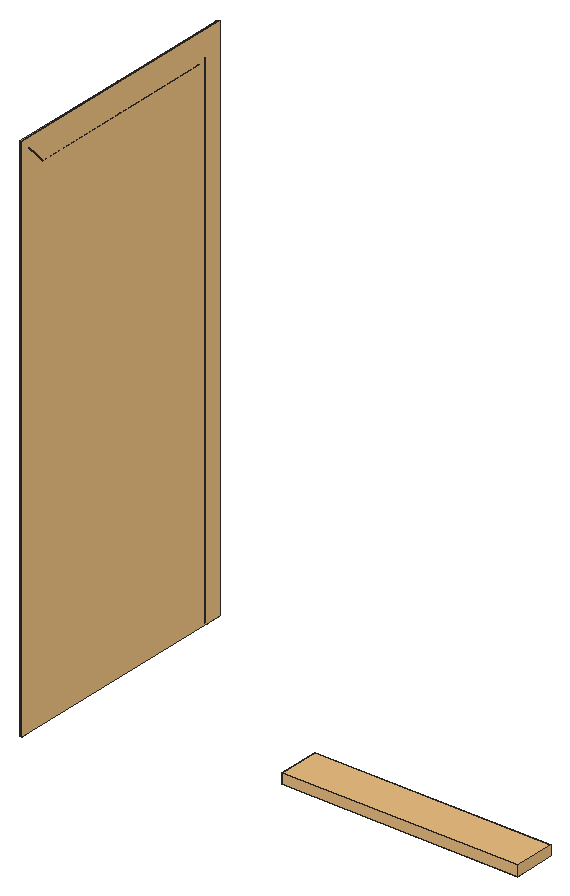
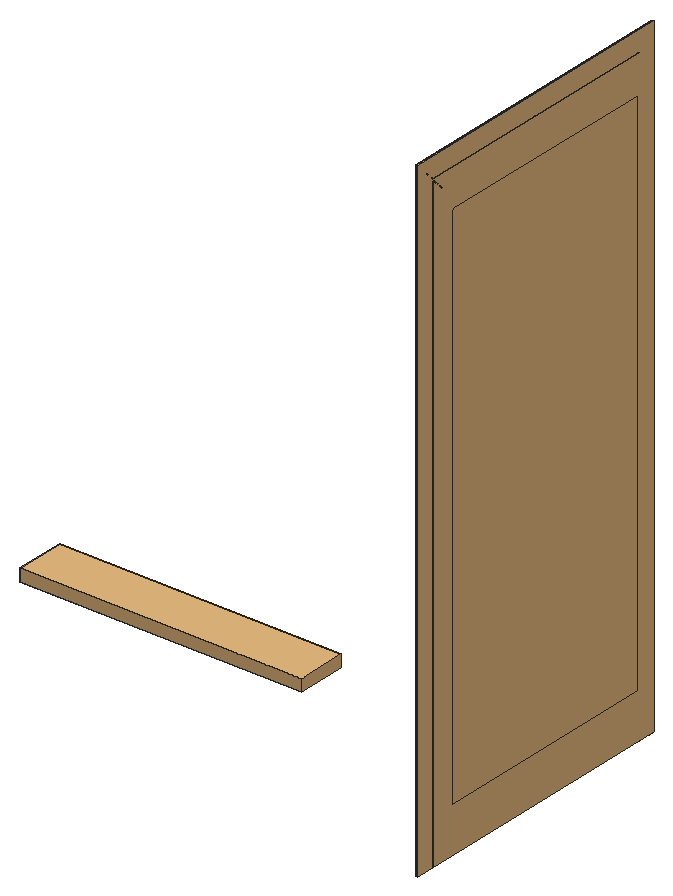
# SketchUp Ruby script. Lengths in inches.
U = 1.inch
M = Sketchup.active_model
def pt(a) = Geom::Point3d.new(a.map { |v| v * U })
def face(e, loops, mat)
  f = e.add_face(loops[0].map { |a| pt(a) })
  loops[1..].each { |l| e.add_face(l.map { |a| pt(a) }).erase! }
  f.material = f.back_material = mat if mat
  f
end
# faces: each face lists its corners as indices into pts; further lists are holes
def faces(e, pts, list, mat = nil) = list.each { |f| face(e, (f[0].is_a?(Array) ? f : [f]).map { |l| l.map { |i| pts[i] } }, mat) }
# xy, xz, yz: faces in a plane at the given z, y or x. An outline is a flat list of corners, or four numbers for a rectangle; further outlines are holes
def ring(l) = l.size == 4 ? [[l[0], l[1]], [l[2], l[1]], [l[2], l[3]], [l[0], l[3]]] : l.each_slice(2).to_a
def flat(e, list, mat, &to3) = list.each { |f| face(e, (f[0].is_a?(Array) ? f : [f]).map { |l| ring(l).map { |u, v| to3.(u, v) } }, mat) }
def xy(e, z, list, mat = nil) = flat(e, list, mat) { |x, y| [x, y, z] }
def xz(e, y, list, mat = nil) = flat(e, list, mat) { |x, z| [x, y, z] }
def yz(e, x, list, mat = nil) = flat(e, list, mat) { |y, z| [x, y, z] }
def lines(e, pts, list) = list.each { |a, b| e.add_line(pt(pts[a]), pt(pts[b])) }
# prism: a flat outline (further loops are holes) pulled along v
def prism(e, loops, v, mat = nil)
  f = face(e, loops, mat); d = Geom::Vector3d.new(v.map { |x| x * U })
  f.pushpull(f.normal.samedirection?(d) ? d.length : -d.length)
end
def box(e, o, s, mat = nil) = prism(e, [[o, [o[0] + s[0], o[1], o[2]], [o[0] + s[0], o[1] + s[1], o[2]], [o[0], o[1] + s[1], o[2]]]], [0, 0, s[2]], mat)
def at(x, y, z, deg = 0) = Geom::Transformation.translation(pt([x, y, z])) * Geom::Transformation.rotation(ORIGIN, Z_AXIS, deg.degrees)
def axes(o, x, y, z) = Geom::Transformation.new([*x, 0, *y, 0, *z, 0, *pt(o).to_a, 1])
def part(name) = M.definitions.add(name)
# library, detail: a bought-in or finely detailed component or shape, given as its bounding box
def library(name, o, s) = part(name).tap { |d| box(d.entities, o, s) }
def detail(e, o, s) = box(e.add_group.entities, o, s)
def put(e, d, t, mat = nil) = e.add_instance(d, t).tap { |i| i.material = mat if mat }
def group(e, t, mat = nil) = e.add_group.tap { |g| g.transformation = t; g.material = mat if mat }.entities
root = M.entities
M.materials.add("Material \#0").color = [86, 53, 35]
M.materials.add("Material \#1").color = [140, 140, 140]
c1 = library("3DGeom~7_Defintion",[455.56,-471.94,-18.85],[5.55,1000,5.48])
c2 = library("3DGeom~9_Defintion",[456.52,-471.89,-18.89],[5.57,1000,5.49])
c3 = library("bedroom2",[0.875,0,0],[46.66,8.22,2])
c4 = library("3DGeom~6_Defintion",[-5.59,-471.8,-48.03],[468.87,1000,73.72])
c5 = part("3DGeom~17_Defintion")
yz(c5.entities,-1908.8,[[-436.03,-21.87,-436.73,-21.5,-435.91,-21.83],[436.03,-21.87,435.91,-21.83,436.73,-21.5],[-435.91,-21.83,-436.73,-21.5,-436.15,-21.125],[-435.91,-21.83,-436.15,-21.125,-435.87,-21.72],[435.91,-21.83,435.87,-21.72,436.15,-21.125],
  [435.91,-21.83,436.15,-21.125,436.73,-21.5],[-436.73,-21.5,-484.73,-21.37,-436.15,-1.11],[-471.46,-21.5,-484.73,-21.37,-436.73,-21.5],[-477.2,-21.5,-484.73,-21.37,-471.46,-21.5],[-481.82,-21.5,-484.73,-21.37,-477.2,-21.5],
  [-436.73,-21.5,-436.15,-1.11,-436.15,-21.125],[436.73,-21.5,436.15,-21.125,471.46,-21.5],[471.46,-21.5,436.15,-21.125,477.2,-21.5],[477.2,-21.5,436.15,-21.125,499.98,-0.85],[477.2,-21.5,499.98,-0.85,481.82,-21.5],
  [481.82,-21.5,487.35,-21,484.73,-21.37],[481.82,-21.5,491.8,-19.52,487.35,-21],[481.82,-21.5,497.64,-13.67,491.8,-19.52],[481.82,-21.5,499.98,-0.85,497.64,-13.67],[-484.73,-21.37,-498.5,-11.58,-499.84,-0.37],
  [-484.73,-21.37,-499.84,-0.37,-499.4,-0.5],[-484.73,-21.37,-499.4,-0.5,-436.15,-1.11],[-484.73,-21.37,-493.63,-18.42,-498.5,-11.58],[-484.73,-21.37,-489.71,-20.375,-493.63,-18.42],[-484.73,-21.37,-487.35,-21,-489.71,-20.375],
  [436.15,-21.125,436.15,-1.11,436.73,-0.74],[436.15,-21.125,436.73,-0.74,499.98,-0.85],[487.35,-21,491.8,-19.52,489.71,-20.375],[-489.71,-20.375,-491.8,-19.52,-493.63,-18.42],[491.8,-19.52,495.21,-17.08,493.63,-18.42],
  [491.8,-19.52,497.64,-13.67,495.21,-17.08],[-493.63,-18.42,-496.54,-15.5,-498.5,-11.58],[-493.63,-18.42,-495.21,-17.08,-496.54,-15.5],[495.21,-17.08,497.64,-13.67,496.54,-15.5],[-496.54,-15.5,-497.64,-13.67,-498.5,-11.58],
  [497.64,-13.67,499.125,-9.22,498.5,-11.58],[497.64,-13.67,499.625,-3.69,499.125,-9.22],[497.64,-13.67,499.98,-0.85,499.625,-3.69],[-498.5,-11.58,-499.625,-3.69,-499.84,-0.37],[-498.5,-11.58,-499.5,-6.6,-499.625,-3.69],
  [-498.5,-11.58,-499.125,-9.22,-499.5,-6.6],[499.125,-9.22,499.625,-3.69,499.5,-6.6],[-499.625,-3.69,-499.98,-0.85,-500,-0.52],[-499.625,-3.69,-500,-0.52,-499.84,-0.37],[-436.15,-1.11,-499.4,-0.5,-471.46,-0.74],
  [-436.15,-1.11,-471.46,-0.74,-436.73,-0.74],[-436.15,-1.11,-436.73,-0.74,-435.91,-0.41],[-436.15,-1.11,-435.91,-0.41,-435.87,-0.52],[436.15,-1.11,435.87,-0.52,435.91,-0.41],[436.15,-1.11,435.91,-0.41,436.73,-0.74],
  [499.98,-0.85,436.73,-0.74,471.46,-0.74],[499.98,-0.85,471.46,-0.74,499.4,-0.5],[499.98,-0.85,499.4,-0.5,499.96,-0.41],[499.98,-0.85,499.96,-0.41,500,-0.52],[-436.73,-0.74,-436.03,-0.37,-435.91,-0.41],
  [436.73,-0.74,435.91,-0.41,436.03,-0.37],[-500,-0.52,-499.96,-0.41,-499.84,-0.37],[499.4,-0.5,499.84,-0.37,499.96,-0.41],[-499.84,141.21,-499.96,141.25,-499.4,141.35],[-436.03,141.21,-436.73,141.59,-435.91,141.25],
  [436.03,141.21,435.91,141.25,436.73,141.59],[499.84,141.21,484.73,162.21,498.5,152.42],[499.84,141.21,499.4,141.35,484.73,162.21],[499.84,141.21,498.5,152.42,499.625,144.53],[499.84,141.21,499.625,144.53,500,141.37],
  [499.84,141.21,500,141.37,499.96,141.25],[-499.96,141.25,-500,141.37,-499.98,141.69],[-499.96,141.25,-499.98,141.69,-499.4,141.35],[-435.91,141.25,-436.73,141.59,-436.15,141.96],[-435.91,141.25,-436.15,141.96,-435.87,141.37],
  [435.91,141.25,435.87,141.37,436.15,141.96],[435.91,141.25,436.15,141.96,436.73,141.59],[-499.4,141.35,-499.98,141.69,-471.46,141.59],[499.4,141.35,436.15,141.96,484.73,162.21],[499.4,141.35,471.46,141.59,436.15,141.96],
  [500,141.37,499.625,144.53,499.98,141.69],[-436.73,141.59,-499.98,141.69,-436.15,161.97],[-471.46,141.59,-499.98,141.69,-436.73,141.59],[-436.73,141.59,-436.15,161.97,-436.15,141.96],[436.73,141.59,436.15,141.96,471.46,141.59],
  [-499.98,141.69,-477.2,162.34,-436.15,161.97],[-499.98,141.69,-481.82,162.34,-477.2,162.34],[-499.98,141.69,-497.64,154.51,-481.82,162.34],[-499.98,141.69,-499.625,144.53,-497.64,154.51],[436.15,141.96,436.15,161.97,436.73,162.34],
  [436.15,141.96,436.73,162.34,484.73,162.21],[-499.625,144.53,-499.125,150.07,-497.64,154.51],[-499.625,144.53,-499.5,147.44,-499.125,150.07],[499.625,144.53,498.5,152.42,499.5,147.44],[499.5,147.44,498.5,152.42,499.125,150.07],
  [-499.125,150.07,-498.5,152.42,-497.64,154.51],[498.5,152.42,484.73,162.21,493.63,159.26],[498.5,152.42,493.63,159.26,496.54,156.34],[498.5,152.42,496.54,156.34,497.64,154.51],[-497.64,154.51,-491.8,160.36,-481.82,162.34],
  [-497.64,154.51,-495.21,157.92,-491.8,160.36],[-497.64,154.51,-496.54,156.34,-495.21,157.92],[496.54,156.34,493.63,159.26,495.21,157.92],[-495.21,157.92,-493.63,159.26,-491.8,160.36],[493.63,159.26,484.73,162.21,489.71,161.22],
  [493.63,159.26,489.71,161.22,491.8,160.36],[-491.8,160.36,-487.35,161.84,-481.82,162.34],[-491.8,160.36,-489.71,161.22,-487.35,161.84],[489.71,161.22,484.73,162.21,487.35,161.84],[-487.35,161.84,-484.73,162.21,-481.82,162.34],
  [-436.15,161.97,-477.2,162.34,-471.46,162.34],[-436.15,161.97,-471.46,162.34,-436.73,162.34],[-436.15,161.97,-436.73,162.34,-435.91,162.68],[-436.15,161.97,-435.91,162.68,-435.87,162.56],[436.15,161.97,435.87,162.56,435.91,162.68],
  [436.15,161.97,435.91,162.68,436.73,162.34],[484.73,162.21,436.73,162.34,471.46,162.34],[484.73,162.21,471.46,162.34,477.2,162.34],[484.73,162.21,477.2,162.34,481.82,162.34],[-436.73,162.34,-436.03,162.72,-435.91,162.68],
  [436.73,162.34,435.91,162.68,436.03,162.72]],"Material \#0")
c6 = library("3DGeom~16_Defintion",[-962.62,-252.34,-11.22],[1000,504.68,93.46])
c7 = part("3DGeom~15_Defintion")
xy(c7.entities,0,[[-961.58,-251.9,-958.5,-248.8125,-961.58,-237.8],[-961.58,-251.9,28.8,-248.8125,-958.5,-248.8125],[-961.58,-251.9,36.25,-251.9,28.8,-248.8125],[36.25,-251.9,19.98,-239.99,28.8,-248.8125],[36.25,-251.9,22.16,-237.8,19.98,-239.99],
  [-958.5,-248.8125,-958.5,-237.8,-961.58,-237.8],[19.98,-239.99,22.16,-237.8,3.36,-223.37],[-958.5,-237.8,-958.5,-223.37,-961.58,-220.28],[-961.58,-237.8,-958.5,-237.8,-961.58,-220.28],[22.16,-237.8,4.64,-220.28,3.36,-223.37],
  [-958.5,-223.37,4.64,-220.28,-961.58,-220.28],[-958.5,-223.37,3.36,-223.37,4.64,-220.28],[5.29,-219.63,8.375,-218.35,5.29,0],[8.375,-218.35,8.375,0,5.29,0],[5.29,0,8.375,0,5.29,219.63],
  [8.375,0,8.375,218.35,5.29,219.63],[8.375,218.35,22.8125,237.15,5.29,219.63],[-961.58,220.28,-958.5,223.37,-961.58,237.8],[-961.58,220.28,3.36,223.37,-958.5,223.37],[-961.58,220.28,4.64,220.28,3.36,223.37],
  [4.64,220.28,19.98,239.99,3.36,223.37],[4.64,220.28,22.16,237.8,19.98,239.99],[-958.5,223.37,-958.5,237.8,-961.58,237.8],[-958.5,237.8,-958.5,248.8125,-961.58,251.9],[-961.58,237.8,-958.5,237.8,-961.58,251.9],
  [22.16,237.8,28.8,248.8125,19.98,239.99],[22.16,237.8,36.25,251.9,28.8,248.8125],[-958.5,248.8125,36.25,251.9,-961.58,251.9],[-958.5,248.8125,28.8,248.8125,36.25,251.9]],"Material \#0")
xy(c7.entities,7.48,[[-962.79,-238.36,23.37,-238.36,-962.79,-219.67],[23.37,-238.36,4.67,-219.67,-962.79,-219.67],[23.37,-238.36,23.37,0,4.67,-219.67],[4.67,-219.67,23.37,0,4.67,0],[23.37,0,23.37,238.36,4.67,219.67],
  [4.67,0,23.37,0,4.67,219.67],[-962.79,219.67,23.37,238.36,-962.79,238.36],[-962.79,219.67,4.67,219.67,23.37,238.36]],"Material \#0")
xy(c7.entities,63.5625,[[-962.79,-238.36,-962.79,-219.67,4.67,-219.67],[-962.79,-238.36,4.67,-219.67,23.37,-238.36],[23.37,-238.36,4.67,-219.67,23.37,0],[4.67,-219.67,4.67,0,23.37,0],[23.37,0,4.67,219.67,23.37,238.36],
  [4.67,0,4.67,219.67,23.37,0],[-962.79,219.67,-962.79,238.36,4.67,219.67],[4.67,219.67,-962.79,238.36,23.37,238.36]],"Material \#0")
xy(c7.entities,69.64,[[-962.79,-219.62,4.63,-219.62,-962.79,-200.32],[4.63,-219.62,-14.68,-200.32,-962.79,-200.32],[4.63,-219.62,4.63,0,-14.68,-200.32],[-14.68,-200.32,4.63,0,-14.68,0],[-14.68,0,4.63,0,-14.68,200.32],
  [4.63,0,4.63,219.62,-14.68,200.32],[-962.79,200.32,-14.68,200.32,4.63,219.62],[-962.79,200.32,4.63,219.62,-962.79,219.62]],"Material \#0")
xy(c7.entities,71.04,[[-961.58,-251.9,-958.5,-248.8125,28.8,-248.8125],[-961.58,-251.9,-961.58,-237.8,-958.5,-248.8125],[-961.58,-251.9,28.8,-248.8125,36.25,-251.9],[36.25,-251.9,19.98,-239.99,22.16,-237.8],[36.25,-251.9,28.8,-248.8125,19.98,-239.99],
  [-958.5,-248.8125,-961.58,-237.8,-958.5,-237.8],[19.98,-239.99,3.36,-223.37,22.16,-237.8],[-958.5,-237.8,-961.58,-220.28,-958.5,-223.37],[-961.58,-237.8,-961.58,-220.28,-958.5,-237.8],[22.16,-237.8,3.36,-223.37,4.64,-220.28],
  [-958.5,-223.37,-961.58,-220.28,4.64,-220.28],[-958.5,-223.37,4.64,-220.28,3.36,-223.37],[5.29,-219.63,5.29,0,8.375,-218.35],[8.375,-218.35,5.29,0,8.375,0],[5.29,0,5.29,219.63,8.375,0],
  [8.375,0,5.29,219.63,8.375,218.35],[8.375,218.35,5.29,219.63,22.8125,237.15],[-961.58,220.28,-958.5,223.37,3.36,223.37],[-961.58,220.28,-961.58,237.8,-958.5,223.37],[-961.58,220.28,3.36,223.37,4.64,220.28],
  [4.64,220.28,3.36,223.37,19.98,239.99],[4.64,220.28,19.98,239.99,22.16,237.8],[-958.5,223.37,-961.58,237.8,-958.5,237.8],[-958.5,237.8,-961.58,251.9,-958.5,248.8125],[-961.58,237.8,-961.58,251.9,-958.5,237.8],
  [22.16,237.8,19.98,239.99,28.8,248.8125],[22.16,237.8,28.8,248.8125,36.25,251.9],[-958.5,248.8125,-961.58,251.9,36.25,251.9],[-958.5,248.8125,36.25,251.9,28.8,248.8125]],"Material \#0")
xz(c7.entities,-238.36,[[-962.79,63.5625,23.37,63.5625,23.37,72.07],[-962.79,63.5625,23.37,72.07,-962.79,72.07]],"Material \#0")
xz(c7.entities,-219.67,[[-962.79,7.48,4.67,7.48,-962.79,63.5625],[4.67,7.48,4.67,63.5625,-962.79,63.5625]],"Material \#0")
xz(c7.entities,219.67,[[-962.79,7.48,-962.79,63.5625,4.67,7.48],[4.67,7.48,-962.79,63.5625,4.67,63.5625]],"Material \#0")
xz(c7.entities,238.36,[[-962.79,63.5625,-962.79,72.07,23.37,72.07],[-962.79,63.5625,23.37,72.07,23.37,63.5625]],"Material \#0")
yz(c7.entities,4.67,[[-219.67,7.48,0,7.48,-219.67,63.5625],[0,7.48,0,63.5625,-219.67,63.5625],[0,7.48,219.67,63.5625,0,63.5625],[0,7.48,219.67,7.48,219.67,63.5625]],"Material \#0")
yz(c7.entities,23.37,[[-238.36,63.5625,0,63.5625,-238.36,72.07],[0,63.5625,0,72.07,-238.36,72.07],[0,63.5625,238.36,63.5625,238.36,72.07],[0,63.5625,238.36,72.07,0,72.07]],"Material \#0")
p = [[36.9,-251.24,0],[37.21,0,-0.16],[34.125,0,-0.14],[36.9,251.24,0],[33.83,243.81,0.02],[33.83,-243.8,0.02],
  [22.8125,-237.15,0],[24.99,-234.97,-0.01],[5.375,-220.37,0],[23.37,-238.36,7.48],[4.67,-219.67,7.48],[4.67,-219.67,7.48],
  [23.37,-238.36,7.48],[23.37,-238.36,0],[4.67,-219.67,7.48],[23.37,-238.36,0],[5.375,-220.37,0],[5.375,-220.37,0],
  [23.37,-238.36,0],[5.29,-219.63,0],[8.375,-218.35,0],[-15.36,-199.64,1.62],[4.67,-219.67,7.48],[5.375,-220.37,0],
  [-13.8,-201.19,0.06],[5.375,-220.37,0],[5.375,-220.37,0],[-14.84,-200.15,0.58],[5.375,-220.37,0],[-13.8,-201.19,0.06],
  [-6.08,-208.92,0],[5.375,-220.37,0],[-13.8,-201.19,0.06],[-6.08,-208.92,0],[-13.8,-201.19,0.06],[5.375,-220.37,0],
  [-6.08,-208.92,0],[-13.8,-201.19,0.06],[-13.09,-201.91,0],[-6.08,-208.92,0],[-13.09,-201.91,0],[-13.8,-201.19,0.06],
  [-15.36,199.64,1.62],[4.67,219.67,7.48],[5.375,220.37,0],[-13.8,201.19,0.06],[5.375,220.37,0],[5.375,220.37,0],
  [4.67,219.67,7.48],[-14.84,200.15,0.58],[5.375,220.37,0],[-13.8,201.19,0.06],[-6.08,208.92,0],[-13.09,201.91,0],
  [-13.8,201.19,0.06],[-6.08,208.92,0],[-13.8,201.19,0.06],[5.375,220.37,0],[-6.08,208.92,0],[5.375,220.37,0],
  [-13.8,201.19,0.06],[-6.08,208.92,0],[-13.8,201.19,0.06],[-13.09,201.91,0],[8.375,218.35,0],[24.99,234.97,-0.01],
  [22.8125,237.15,0],[23.37,238.36,7.48],[23.37,238.36,0],[23.37,238.36,0],[5.375,220.37,0],[5.375,220.37,0],
  [23.37,238.36,7.48],[4.67,219.67,7.48],[5.375,220.37,0],[23.37,238.36,0],[23.37,238.36,7.48],[-13.8,-201.19,0.06],
  [-14.84,-200.15,0.58],[-14.38,-200.61,0.26],[-13.8,-201.19,0.06],[-13.8,-201.19,0.06],[-14.38,-200.61,0.26],[-13.8,201.19,0.06],
  [-14.84,200.15,0.58],[-13.8,201.19,0.06],[-14.38,200.61,0.26],[-14.38,200.61,0.26],[-13.8,201.19,0.06],[4.63,-219.62,69.64],
  [4.63,-219.62,69.64],[-15.42,-199.57,9.43],[-15.36,-199.64,1.62],[-15.16,-199.83,1.04],[-15.16,-199.83,1.04],[-15.16,199.83,1.04],
  [-15.36,199.64,1.62],[-15.16,199.83,1.04],[-15.42,199.57,9.43],[4.63,219.62,69.64],[4.67,219.67,7.48],[4.63,219.62,69.64],
  [4.63,-219.62,69.64],[4.67,-219.67,63.5625],[4.67,-219.67,63.5625],[4.67,-219.67,7.48],[-15.28,-199.71,69.25],[4.63,-219.62,69.64],
  [-15.42,-199.57,9.43],[-15.28,-199.71,69.25],[-15.42,-199.57,2.34],[-15.42,-199.57,2.34],[-15.42,199.57,2.34],[-15.42,199.57,9.43],
  [-15.28,199.71,69.25],[-15.28,199.71,69.25],[4.63,219.62,69.64],[4.63,219.62,69.64],[4.67,219.67,63.5625],[4.67,219.67,63.5625],
  [-15.42,199.57,2.34],[4.67,-219.67,63.5625],[4.63,-219.62,69.64],[4.67,219.67,7.48],[4.67,219.67,63.5625],[4.63,219.62,69.64],
  [4.63,-219.62,69.64],[-15.28,-199.71,69.25],[-15.28,-199.71,69.25],[-15.42,-199.57,48.99],[-15.42,-199.57,48.99],[-15.28,-199.71,69.25],
  [-15.42,199.57,48.99],[-15.28,199.71,69.25],[-15.28,199.71,69.25],[-15.42,199.57,48.99],[4.63,219.62,69.64],[4.63,-219.62,69.64],
  [23.37,-238.36,72.07],[4.67,-219.67,63.5625],[4.67,-219.67,63.5625],[23.37,-238.36,63.5625],[23.37,-238.36,72.07],[4.67,-219.67,63.5625],
  [5.24,-220.23,70.03],[23.37,-238.36,72.07],[23.37,-238.36,63.5625],[4.67,-219.67,63.5625],[4.67,-219.67,63.5625],[4.63,-219.62,69.64],
  [4.63,219.62,69.64],[23.37,238.36,72.07],[4.67,219.67,63.5625],[4.67,219.67,63.5625],[5.24,220.23,70.03],[4.63,219.62,69.64],
  [23.37,238.36,63.5625],[4.67,219.67,63.5625],[4.67,219.67,63.5625],[23.37,238.36,63.5625],[23.37,238.36,72.07],[4.67,219.67,63.5625],
  [23.37,238.36,72.07],[4.63,-219.62,69.64],[-14.68,-200.32,69.64],[-15.28,-199.71,69.25],[-15.28,-199.71,69.25],[-14.68,-200.32,69.64],
  [4.63,-219.62,69.64],[-15.28,199.71,69.25],[-14.68,200.32,69.64],[4.63,219.62,69.64],[4.63,219.62,69.64],[-14.68,200.32,69.64],
  [4.63,-219.62,69.64],[5.24,-220.23,70.03],[23.37,-238.36,72.07],[4.63,219.62,69.64],[5.24,220.23,70.03],[5.375,-220.37,72.07],
  [5.375,-220.37,72.07],[23.37,-238.36,72.07],[5.375,220.37,72.07],[23.37,238.36,72.07],[5.375,220.37,72.07],[33.83,-243.8,71.03],
  [36.9,-251.24,71.04],[22.8125,-237.15,71.04],[34.125,0,71.19],[37.21,0,71.2],[24.99,-234.97,71.05],[5.29,-219.63,71.04],
  [8.375,-218.35,71.04],[33.83,243.81,71.03],[36.9,251.24,71.04],[22.8125,237.15,71.04],[24.99,234.97,71.05],[8.375,218.35,71.04]]
faces(c7.entities,p,[[0,1,2],[1,3,4],[4,2,1],[2,5,0],[6,0,5],[5,7,6],[8,9,10],[11,12,13],
  [14,15,16],[17,18,9],[19,6,7],[7,20,19],[21,22,23],[24,21,25],[26,10,27],[28,27,29],
  [30,31,32],[33,34,35],[36,37,38],[39,40,41],[42,43,44],[45,42,46],[47,48,49],[50,49,51],
  [52,53,54],[55,56,57],[58,59,60],[61,62,63],[64,65,66],[43,67,68],[43,69,70],[71,72,73],
  [74,75,76],[3,66,65],[65,4,3],[77,78,21],[27,79,80],[81,82,78],[83,84,42],[85,86,84],
  [49,87,88],[10,89,27],[90,91,27],[92,93,27],[91,92,27],[78,94,21],[84,95,42],[96,97,49],
  [98,96,49],[99,98,49],[100,101,49],[21,102,103],[21,104,105],[21,106,107],[21,108,109],[91,110,92],
  [21,111,108],[42,112,113],[42,113,114],[42,115,116],[42,117,118],[42,119,43],[98,120,96],[10,121,122],
  [123,124,125],[126,127,91],[128,129,91],[108,130,131],[113,132,133],[134,135,98],[136,134,98],[137,138,139],
  [140,141,142],[143,142,144],[145,146,147],[148,144,149],[150,151,152],[153,154,155],[151,156,157],[158,159,160],
  [161,162,154],[163,164,165],[166,167,168],[169,170,171],[172,173,134],[174,175,176],[177,178,151],[142,179,144],
  [175,180,181],[178,182,151],[183,184,154],[185,186,187],[186,185,188],[188,189,186],[187,190,185],[190,187,191],
  [191,192,190],[189,188,193],[193,194,189],[195,196,197],[196,195,194],[194,193,196]],"Material \#0")
c8 = part("3DGeom~19_Defintion")
xy(c8.entities,0,[[-6.28,-215.79,-994.45,-208.55,-13.52,-208.55],[-994.45,-215.79,-994.45,-208.55,-6.28,-215.79],[-6.28,-215.79,-13.52,-208.55,-13.52,0],[-6.28,-215.79,-13.52,0,-6.28,0],[-13.52,0,-13.52,208.55,-6.28,215.79],
  [-13.52,0,-6.28,215.79,-6.28,0],[-994.45,208.55,-6.28,215.79,-13.52,208.55],[-994.45,208.55,-994.45,215.79,-6.28,215.79]],"Material \#0")
p = [[-13.52,-208.55,0],[-994.45,-208.55,0],[-994.45,-207.81,0.07],[-14.25,-207.81,0.07],[-13.52,-208.55,0],[-14.25,-207.81,0.07],
  [-14.25,0,0.07],[-13.52,0,0],[-13.52,208.55,0],[-14.25,207.81,0.07],[-13.52,208.55,0],[-14.25,207.81,0.07],
  [-994.45,207.81,0.07],[-994.45,208.55,0],[-994.45,-207.21,0.27],[-994.45,-207.21,0.27],[-14.86,-207.21,0.27],[-14.86,-207.21,0.27],
  [-14.86,0,0.27],[-14.86,0,0.27],[-14.86,0,0.27],[-14.86,0,0.27],[-14.86,207.21,0.27],[-14.86,207.21,0.27],
  [-994.45,207.21,0.27],[-994.45,207.21,0.27],[-14.86,-207.21,0.27],[-994.45,-207.21,0.27],[-994.45,-206.74,0.6],[-15.33,-206.74,0.6],
  [-14.86,-207.21,0.27],[-15.33,-206.74,0.6],[-15.33,0,0.6],[-14.86,0,0.27],[-14.86,207.21,0.27],[-15.33,206.74,0.6],
  [-14.86,207.21,0.27],[-15.33,206.74,0.6],[-994.45,206.74,0.6],[-994.45,207.21,0.27],[-994.45,-206.4,1.07],[-15.66,-206.4,1.07],
  [-15.66,-206.4,1.07],[-15.66,0,1.07],[-15.66,206.4,1.07],[-15.66,206.4,1.07],[-994.45,206.4,1.07],[-994.45,-206.2,1.68],
  [-15.86,-206.2,1.68],[-15.86,-206.2,1.68],[-15.86,0,1.68],[-15.86,206.2,1.68],[-15.86,206.2,1.68],[-994.45,206.2,1.68],
  [-994.45,-206.13,2.41],[-15.93,-206.13,2.41],[-15.93,-206.13,2.41],[-15.93,0,2.41],[-15.93,206.13,2.41],[-15.93,206.13,2.41],
  [-994.45,206.13,2.41],[-994.45,-206.13,71.16],[-994.45,-206.22,71.59],[-15.79,-206.28,71.53],[-15.79,-206.28,71.53],[-15.84,0,71.59],
  [-15.93,0,71.16],[-15.79,206.28,71.53],[-15.79,206.28,71.53],[-994.45,206.22,71.59],[-994.45,206.13,71.16],[-15.79,-206.28,71.53],
  [-994.45,-206.48,71.84],[-994.45,-206.9,71.93],[-15.16,-206.9,71.93],[-15.79,-206.28,71.53],[-15.79,-206.28,71.53],[-15.16,-206.9,71.93],
  [-15.16,0,71.93],[-994.45,-206.48,71.84],[-15.59,0,71.84],[-15.79,-206.28,71.53],[-15.59,0,71.84],[-15.79,206.28,71.53],
  [-15.16,206.9,71.93],[-15.59,0,71.84],[-15.79,206.28,71.53],[-994.45,206.48,71.84],[-15.79,206.28,71.53],[-15.16,206.9,71.93],
  [-994.45,206.9,71.93],[-994.45,206.48,71.84],[-15.79,206.28,71.53],[-994.45,-227.27,72.01],[5.41,-227.47,72.33],[4.78,-226.84,71.93],
  [4.78,-226.84,71.93],[5.41,-227.47,72.33],[5.21,0,72.01],[-994.45,-226.84,71.93],[-994.45,-227.27,72.01],[5.21,0,72.01],
  [4.78,0,71.93],[4.78,226.84,71.93],[5.21,0,72.01],[5.21,0,72.01],[5.41,227.47,72.33],[4.78,226.84,71.93],
  [5.41,227.47,72.33],[-994.45,227.27,72.01],[-994.45,227.27,72.01],[-994.45,226.84,71.93],[-994.45,-227.27,72.01],[-994.45,-227.53,72.27],
  [5.41,-227.47,72.33],[5.41,-227.47,72.33],[5.47,0,72.27],[5.21,0,72.01],[5.41,227.47,72.33],[5.41,227.47,72.33],
  [-994.45,227.53,72.27],[-994.45,227.27,72.01],[-994.45,-227.61,72.7],[-994.45,-227.61,74.4375],[-994.45,-227.61,74.4375],[5.55,-227.61,74.4375],
  [5.55,-227.61,74.4375],[5.55,0,74.4375],[5.55,0,72.7],[5.55,227.61,74.4375],[5.55,227.61,74.4375],[-994.45,227.61,74.4375],
  [-994.45,227.61,74.4375],[-994.45,227.61,72.7]]
faces(c8.entities,p,[[0,1,2],[2,3,0],[4,5,6],[6,7,4],[8,7,6],[6,9,8],[10,11,12],[12,13,10],
  [3,2,14],[15,16,3],[5,17,18],[19,6,5],[9,6,20],[21,22,9],[11,23,24],[25,12,11],
  [26,27,28],[28,29,26],[30,31,32],[32,33,30],[34,33,32],[32,35,34],[36,37,38],[38,39,36],
  [29,28,40],[40,41,29],[31,42,43],[43,32,31],[35,32,43],[43,44,35],[37,45,46],[46,38,37],
  [41,40,47],[47,48,41],[42,49,50],[50,43,42],[44,43,50],[50,51,44],[45,52,53],[53,46,45],
  [48,47,54],[54,55,48],[49,56,57],[57,50,49],[51,50,57],[57,58,51],[52,59,60],[60,53,52],
  [61,62,63],[64,65,66],[66,65,67],[68,69,70],[71,72,73],[73,74,75],[76,77,78],[62,79,63],
  [78,80,76],[81,82,65],[83,80,78],[78,84,83],[65,85,86],[68,87,69],[88,89,90],[90,91,92],
  [93,94,95],[96,97,98],[95,99,100],[101,102,96],[103,102,104],[105,106,103],[107,108,109],[110,111,107],
  [112,113,114],[115,116,117],[117,116,118],[119,120,121],[114,122,123],[124,125,114],[113,122,114],[115,126,127],
  [127,128,115],[115,128,116],[118,128,127],[127,129,118],[116,128,118],[119,130,131],[132,133,119],[119,133,120]],"Material \#0")
xy(root,7.655,[[362.607,164.24,362.604,164.254,362.604,164.275],[362.607,164.24,362.604,164.275,362.607,164.263],[362.607,164.24,362.607,164.263,362.611,164.254],[362.604,164.254,362.601,164.293,362.601,164.31],[362.604,164.254,362.601,164.31,362.604,164.275],
  [362.611,164.254,362.607,164.263,362.61,164.275],[362.611,164.254,362.61,164.275,362.614,164.293],[362.61,164.275,362.613,164.31,362.614,164.293],[362.601,164.293,362.598,164.353,362.599,164.365],[362.601,164.293,362.599,164.365,362.601,164.31],
  [362.614,164.293,362.613,164.31,362.616,164.353],[362.613,164.31,362.615,164.365,362.616,164.353],[362.598,164.353,362.597,164.427,362.598,164.431],[362.598,164.353,362.598,164.431,362.599,164.365],[362.616,164.353,362.615,164.365,362.617,164.427],
  [362.615,164.365,362.616,164.431,362.617,164.427],[362.597,164.427,362.597,164.506,362.598,164.502],[362.597,164.427,362.598,164.502,362.598,164.431],[362.617,164.427,362.616,164.431,362.617,164.506],[362.616,164.431,362.616,164.502,362.617,164.506],
  [362.598,164.502,362.597,164.506,362.599,164.568],[362.616,164.502,362.615,164.568,362.616,164.579],[362.616,164.502,362.616,164.579,362.617,164.506],[362.597,164.506,362.598,164.579,362.599,164.568],[362.599,164.568,362.598,164.579,362.601,164.622],
  [362.615,164.568,362.613,164.622,362.614,164.64],[362.615,164.568,362.614,164.64,362.616,164.579],[362.598,164.579,362.601,164.64,362.601,164.622],[362.601,164.622,362.601,164.64,362.604,164.658],[362.613,164.622,362.61,164.658,362.611,164.679],
  [362.613,164.622,362.611,164.679,362.614,164.64],[362.601,164.64,362.604,164.679,362.604,164.658],[362.604,164.658,362.604,164.679,362.607,164.67],[362.61,164.658,362.607,164.67,362.607,164.693],[362.61,164.658,362.607,164.693,362.611,164.679],
  [362.607,164.67,362.604,164.679,362.607,164.693]],"Material \#1")
xy(root,7.675,[[362.607,164.24,362.607,164.263,362.604,164.254],[362.607,164.24,362.61,164.275,362.607,164.263],[362.607,164.24,362.611,164.254,362.61,164.275],[362.604,164.254,362.604,164.275,362.601,164.293],[362.604,164.254,362.607,164.263,362.604,164.275],
  [362.611,164.254,362.613,164.31,362.61,164.275],[362.611,164.254,362.614,164.293,362.613,164.31],[362.604,164.275,362.601,164.31,362.601,164.293],[362.601,164.293,362.601,164.31,362.598,164.353],[362.614,164.293,362.615,164.365,362.613,164.31],
  [362.614,164.293,362.616,164.353,362.615,164.365],[362.601,164.31,362.599,164.365,362.598,164.353],[362.598,164.353,362.599,164.365,362.597,164.427],[362.616,164.353,362.616,164.431,362.615,164.365],[362.616,164.353,362.617,164.427,362.616,164.431],
  [362.599,164.365,362.598,164.431,362.597,164.427],[362.597,164.427,362.598,164.431,362.597,164.506],[362.617,164.427,362.616,164.502,362.616,164.431],[362.617,164.427,362.617,164.506,362.616,164.502],[362.598,164.431,362.598,164.502,362.597,164.506],
  [362.598,164.502,362.598,164.579,362.597,164.506],[362.598,164.502,362.599,164.568,362.598,164.579],[362.616,164.502,362.617,164.506,362.615,164.568],[362.617,164.506,362.616,164.579,362.615,164.568],[362.599,164.568,362.601,164.64,362.598,164.579],
  [362.599,164.568,362.601,164.622,362.601,164.64],[362.615,164.568,362.616,164.579,362.613,164.622],[362.616,164.579,362.614,164.64,362.613,164.622],[362.601,164.622,362.604,164.658,362.604,164.679],[362.601,164.622,362.604,164.679,362.601,164.64],
  [362.613,164.622,362.614,164.64,362.61,164.658],[362.614,164.64,362.611,164.679,362.61,164.658],[362.604,164.658,362.607,164.67,362.607,164.693],[362.604,164.658,362.607,164.693,362.604,164.679],[362.61,164.658,362.611,164.679,362.607,164.67],
  [362.607,164.67,362.611,164.679,362.607,164.693]],"Material \#1")
xy(root,12.098,[[362.607,164.24,362.604,164.254,362.607,164.263],[362.607,164.24,362.607,164.263,362.61,164.275],[362.607,164.24,362.61,164.275,362.611,164.254],[362.604,164.254,362.601,164.293,362.604,164.275],[362.604,164.254,362.604,164.275,362.607,164.263],
  [362.611,164.254,362.61,164.275,362.613,164.31],[362.611,164.254,362.613,164.31,362.614,164.293],[362.604,164.275,362.601,164.293,362.601,164.31],[362.601,164.293,362.598,164.353,362.601,164.31],[362.614,164.293,362.613,164.31,362.615,164.365],
  [362.614,164.293,362.615,164.365,362.616,164.353],[362.601,164.31,362.598,164.353,362.599,164.365],[362.598,164.353,362.597,164.427,362.599,164.365],[362.616,164.353,362.615,164.365,362.616,164.431],[362.616,164.353,362.616,164.431,362.617,164.427],
  [362.599,164.365,362.597,164.427,362.598,164.431],[362.597,164.427,362.597,164.506,362.598,164.431],[362.617,164.427,362.616,164.431,362.616,164.502],[362.617,164.427,362.616,164.502,362.617,164.506],[362.598,164.431,362.597,164.506,362.598,164.502],
  [362.598,164.502,362.597,164.506,362.598,164.579],[362.598,164.502,362.598,164.579,362.599,164.568],[362.616,164.502,362.615,164.568,362.617,164.506],[362.617,164.506,362.615,164.568,362.616,164.579],[362.599,164.568,362.598,164.579,362.601,164.64],
  [362.599,164.568,362.601,164.64,362.601,164.622],[362.615,164.568,362.613,164.622,362.616,164.579],[362.616,164.579,362.613,164.622,362.614,164.64],[362.601,164.622,362.601,164.64,362.604,164.679],[362.601,164.622,362.604,164.679,362.604,164.658],
  [362.613,164.622,362.61,164.658,362.614,164.64],[362.614,164.64,362.61,164.658,362.611,164.679],[362.604,164.658,362.604,164.679,362.607,164.693],[362.604,164.658,362.607,164.693,362.607,164.67],[362.61,164.658,362.607,164.67,362.611,164.679],
  [362.607,164.67,362.607,164.693,362.611,164.679]],"Material \#1")
xy(root,12.118,[[362.607,164.24,362.604,164.275,362.604,164.254],[362.607,164.24,362.607,164.263,362.604,164.275],[362.607,164.24,362.611,164.254,362.607,164.263],[362.604,164.254,362.601,164.31,362.601,164.293],[362.604,164.254,362.604,164.275,362.601,164.31],
  [362.611,164.254,362.61,164.275,362.607,164.263],[362.611,164.254,362.614,164.293,362.61,164.275],[362.61,164.275,362.614,164.293,362.613,164.31],[362.601,164.293,362.599,164.365,362.598,164.353],[362.601,164.293,362.601,164.31,362.599,164.365],
  [362.614,164.293,362.616,164.353,362.613,164.31],[362.613,164.31,362.616,164.353,362.615,164.365],[362.598,164.353,362.598,164.431,362.597,164.427],[362.598,164.353,362.599,164.365,362.598,164.431],[362.616,164.353,362.617,164.427,362.615,164.365],
  [362.615,164.365,362.617,164.427,362.616,164.431],[362.597,164.427,362.598,164.431,362.598,164.502],[362.597,164.427,362.598,164.502,362.597,164.506],[362.617,164.427,362.617,164.506,362.616,164.431],[362.616,164.431,362.617,164.506,362.616,164.502],
  [362.598,164.502,362.599,164.568,362.597,164.506],[362.616,164.502,362.616,164.579,362.615,164.568],[362.616,164.502,362.617,164.506,362.616,164.579],[362.597,164.506,362.599,164.568,362.598,164.579],[362.599,164.568,362.601,164.622,362.598,164.579],
  [362.615,164.568,362.614,164.64,362.613,164.622],[362.615,164.568,362.616,164.579,362.614,164.64],[362.598,164.579,362.601,164.622,362.601,164.64],[362.601,164.622,362.604,164.658,362.601,164.64],[362.613,164.622,362.611,164.679,362.61,164.658],
  [362.613,164.622,362.614,164.64,362.611,164.679],[362.601,164.64,362.604,164.658,362.604,164.679],[362.604,164.658,362.607,164.67,362.604,164.679],[362.61,164.658,362.607,164.693,362.607,164.67],[362.61,164.658,362.611,164.679,362.607,164.693],
  [362.607,164.67,362.607,164.693,362.604,164.679]],"Material \#1")
put(root,c1,axes([362.67,201.8,49.3125],[0,-0.08145,0],[0,0,0.08876],[0.0037,0,0]),"Material \#1")
put(root,c2,axes([362.67,201.8,49.3125],[0,-0.08128,0],[0,0,0.08858],[0.00369,0,0]),"Material \#1")
put(root,c3,at(403.35,173.36,0.5))
put(root,c4,axes([362.67,201.8,49.3125],[0,-0.08102,0],[0,0,0.08829],[0.00368,0,0]),"Material \#1")
put(root,c5,axes([362.93,185.06,101.58],[0,0,0.05322],[0,-0.04883,0],[-0.00222,0,0]),"Material \#0")
put(root,c6,axes([362.93,185.06,101.58],[0,0,0.10553],[0,-0.09684,0],[-0.0044,0,0]),"Material \#0")
put(root,c7,axes([362.93,185.06,101.58],[0,0,0.10551],[0,-0.09682,0],[-0.0044,0,0]),"Material \#0")
put(root,c8,axes([362.93,185.06,101.58],[0,0,0.10215],[0,-0.09374,0],[-0.00426,0,0]),"Material \#0")
